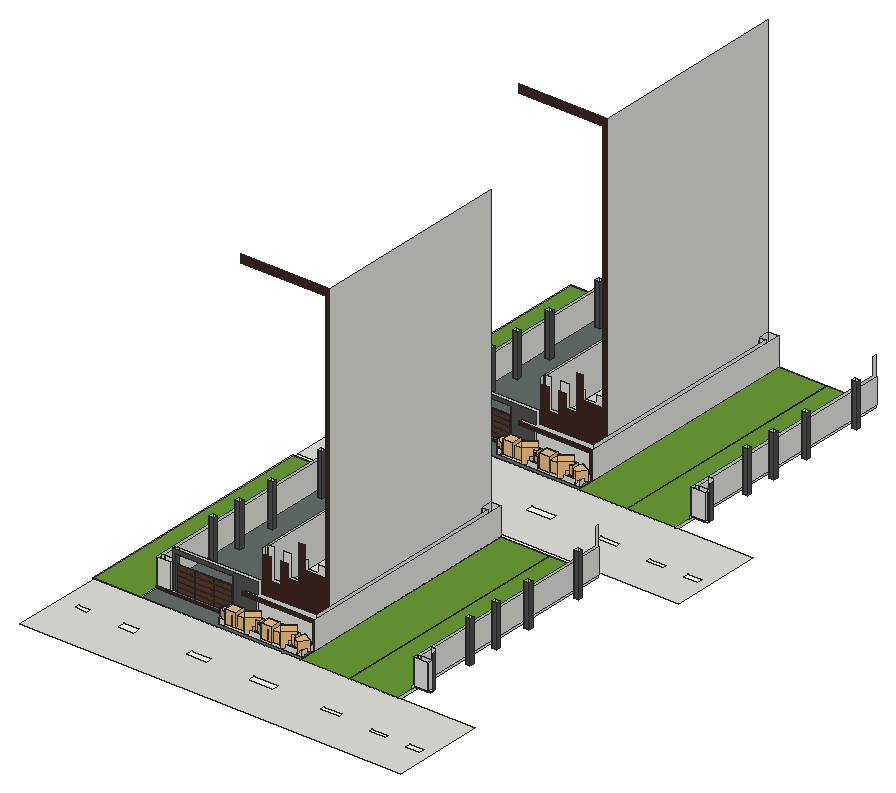
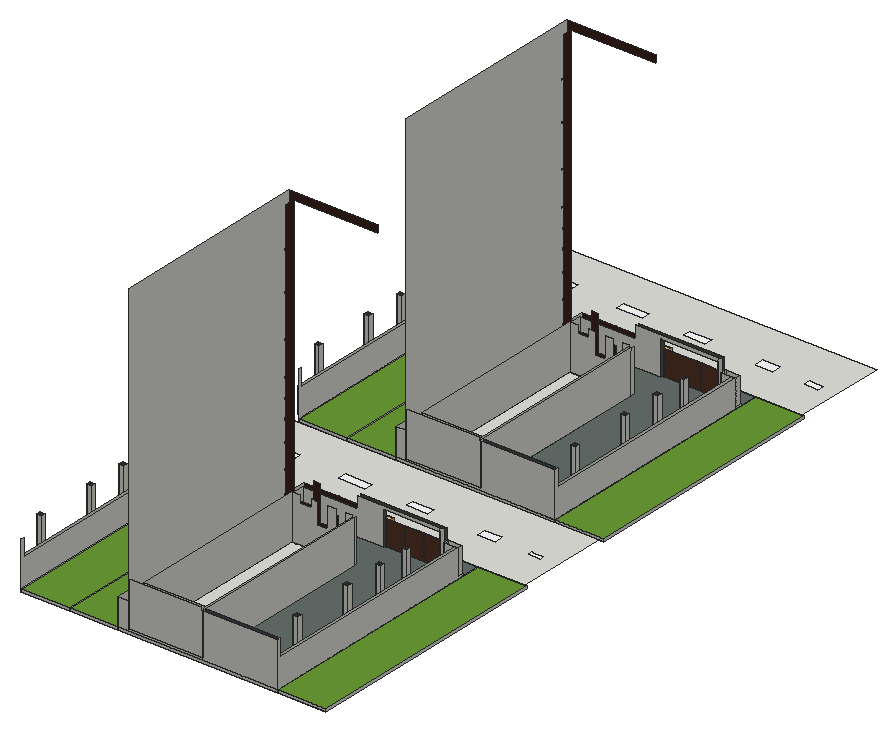
# SketchUp Ruby script. Lengths in inches.
U = 1.inch
M = Sketchup.active_model
def pt(a) = Geom::Point3d.new(a.map { |v| v * U })
def face(e, loops, mat)
  f = e.add_face(loops[0].map { |a| pt(a) })
  loops[1..].each { |l| e.add_face(l.map { |a| pt(a) }).erase! }
  f.material = f.back_material = mat if mat
  f
end
# faces: each face lists its corners as indices into pts; further lists are holes
def faces(e, pts, list, mat = nil) = list.each { |f| face(e, (f[0].is_a?(Array) ? f : [f]).map { |l| l.map { |i| pts[i] } }, mat) }
# xy, xz, yz: faces in a plane at the given z, y or x. An outline is a flat list of corners, or four numbers for a rectangle; further outlines are holes
def ring(l) = l.size == 4 ? [[l[0], l[1]], [l[2], l[1]], [l[2], l[3]], [l[0], l[3]]] : l.each_slice(2).to_a
def flat(e, list, mat, &to3) = list.each { |f| face(e, (f[0].is_a?(Array) ? f : [f]).map { |l| ring(l).map { |u, v| to3.(u, v) } }, mat) }
def xy(e, z, list, mat = nil) = flat(e, list, mat) { |x, y| [x, y, z] }
def xz(e, y, list, mat = nil) = flat(e, list, mat) { |x, z| [x, y, z] }
def yz(e, x, list, mat = nil) = flat(e, list, mat) { |y, z| [x, y, z] }
def lines(e, pts, list) = list.each { |a, b| e.add_line(pt(pts[a]), pt(pts[b])) }
# prism: a flat outline (further loops are holes) pulled along v
def prism(e, loops, v, mat = nil)
  f = face(e, loops, mat); d = Geom::Vector3d.new(v.map { |x| x * U })
  f.pushpull(f.normal.samedirection?(d) ? d.length : -d.length)
end
def box(e, o, s, mat = nil) = prism(e, [[o, [o[0] + s[0], o[1], o[2]], [o[0] + s[0], o[1] + s[1], o[2]], [o[0], o[1] + s[1], o[2]]]], [0, 0, s[2]], mat)
def at(x, y, z, deg = 0) = Geom::Transformation.translation(pt([x, y, z])) * Geom::Transformation.rotation(ORIGIN, Z_AXIS, deg.degrees)
def axes(o, x, y, z) = Geom::Transformation.new([*x, 0, *y, 0, *z, 0, *pt(o).to_a, 1])
def part(name) = M.definitions.add(name)
# library, detail: a bought-in or finely detailed component or shape, given as its bounding box
def library(name, o, s) = part(name).tap { |d| box(d.entities, o, s) }
def detail(e, o, s) = box(e.add_group.entities, o, s)
def put(e, d, t, mat = nil) = e.add_instance(d, t).tap { |i| i.material = mat if mat }
def group(e, t, mat = nil) = e.add_group.tap { |g| g.transformation = t; g.material = mat if mat }.entities
root = M.entities
M.materials.add("Color_").color = [255, 255, 255]
M.materials.add("Material__1").color = [95, 70, 46]
M.materials.add("[0043_SaddleBrown]").color = [63, 38, 31]
M.materials.add("[0135_DarkGray]").color = [81, 81, 81]
M.materials.add("[Color L16]").color = [51, 38, 20]
M.materials.add("[Formica Blue]").color = [73, 80, 86]
M.materials.add("[Grass Dark Green]").color = [105, 155, 54]
M.materials.add("[Slate]").color = [102, 110, 108]
M.materials.add("[Wood Veneer 01]").color = [89, 56, 41]
c1 = part("Grupo\#4")
xy(c1.entities,0,[[0,0,0,3.15,255.91,3.15,255.91,0,171.65,0,171.65,1.57,171.26,1.57,171.26,0,86.22,0,86.22,1.57,85.83,1.57,85.83,0]],"[Wood Veneer 01]")
xy(c1.entities,23.68,[[0,0,85.83,1.57],[86.22,0,171.26,1.57],[171.65,0,186.61,1.57],[186.61,0,255.91,1.57]],"[Color L16]")
xy(c1.entities,24.07,[[0,0,85.83,1.57],[86.22,0,168.11,1.57],[168.11,0,171.26,1.57],[171.65,0,255.91,1.57]],"[Color L16]")
xy(c1.entities,47.3,[[0,0,85.83,1.57],[86.22,0,89.76,1.57],[89.76,0,171.26,1.57],[171.65,0,255.91,1.57]],"[Color L16]")
xy(c1.entities,47.69,[[0,0,85.83,1.57],[86.22,0,171.26,1.57],[171.65,0,255.91,1.57]],"[Color L16]")
xy(c1.entities,70.92,[[0,0,85.83,1.57],[86.22,0,171.26,1.57],[171.65,0,255.91,1.57]],"[Color L16]")
xy(c1.entities,71.3125,[[0,0,85.83,1.57],[86.22,0,171.26,1.57],[171.65,0,255.91,1.57]],"[Color L16]")
xy(c1.entities,94.54,[[0,0,85.83,1.57],[86.22,0,171.26,1.57],[171.65,0,255.91,1.57]],"[Color L16]")
xy(c1.entities,94.9375,[[0,0,85.83,1.57],[86.22,0,171.26,1.57],[171.65,0,255.91,1.57]],"[Color L16]")
xy(c1.entities,118.16,[[0,0,85.83,0,85.83,1.57,86.22,1.57,86.22,0,171.26,0,171.26,1.57,171.65,1.57,171.65,0,255.91,0,255.91,3.15,0,3.15]],"[Wood Veneer 01]")
xz(c1.entities,0,[[0,0,85.83,23.68],[86.22,0,171.26,23.68],[171.65,0,255.91,23.68],[0,24.07,85.83,47.3],[86.22,24.07,171.26,47.3],
  [171.65,24.07,255.91,47.3],[0,47.69,85.83,70.92],[86.22,47.69,171.26,70.92],[171.65,47.69,255.91,70.92],[0,71.3125,85.83,94.54],
  [86.22,71.3125,171.26,94.54],[171.65,71.3125,255.91,94.54],[0,94.9375,85.83,118.16],[86.22,94.9375,171.26,118.16],[171.65,94.9375,255.91,118.16]],"[Wood Veneer 01]")
xz(c1.entities,1.57,[[[85.83,0,86.22,0,86.22,23.68,171.26,23.68,171.26,0,171.65,0,171.65,23.68,255.91,23.68,255.91,24.07,171.65,24.07,171.65,47.3,255.91,47.3,255.91,47.69,171.65,47.69,171.65,70.92,255.91,70.92,255.91,71.3125,171.65,71.3125,171.65,94.54,255.91,94.54,255.91,94.9375,171.65,94.9375,171.65,118.16,171.26,118.16,171.26,94.9375,86.22,94.9375,86.22,118.16,85.83,118.16,85.83,94.9375,0,94.9375,0,94.54,85.83,94.54,85.83,71.3125,0,71.3125,0,70.92,85.83,70.92,85.83,47.69,0,47.69,0,47.3,85.83,47.3,85.83,24.07,0,24.07,0,23.68,85.83,23.68],[86.22,71.3125,171.26,94.54],[86.22,24.07,171.26,47.3],[86.22,47.69,171.26,70.92]]],"[Color L16]")
xz(c1.entities,3.15,[[0,0,255.91,118.16]],"[Wood Veneer 01]")
yz(c1.entities,0,[[0,0,0,23.68,1.57,23.68,1.57,24.07,0,24.07,0,47.3,1.57,47.3,1.57,47.69,0,47.69,0,70.92,1.57,70.92,1.57,71.3125,0,71.3125,0,94.54,1.57,94.54,1.57,94.9375,0,94.9375,0,118.16,3.15,118.16,3.15,0]],"[Wood Veneer 01]")
yz(c1.entities,85.83,[[0,0,1.57,23.68],[0,24.07,1.57,47.3],[0,47.69,1.57,70.92],[0,71.3125,1.57,94.54],[0,94.9375,1.57,118.16]],"[Color L16]")
yz(c1.entities,86.22,[[0,0,1.57,23.68],[0,24.07,1.57,47.3],[0,47.69,1.57,70.92],[0,71.3125,1.57,94.54],[0,94.9375,1.57,118.16]],"[Color L16]")
yz(c1.entities,171.26,[[0,0,1.57,23.68],[0,24.07,1.57,47.3],[0,47.69,1.57,70.92],[0,71.3125,1.57,94.54],[0,94.9375,1.57,118.16]],"[Color L16]")
yz(c1.entities,171.65,[[0,0,1.57,23.68],[0,24.07,1.57,47.3],[0,47.69,1.57,70.92],[0,71.3125,1.57,94.54],[0,94.9375,1.57,118.16]],"[Color L16]")
yz(c1.entities,255.91,[[0,0,3.15,0,3.15,118.16,0,118.16,0,94.9375,1.57,94.9375,1.57,94.54,0,94.54,0,71.3125,1.57,71.3125,1.57,70.92,0,70.92,0,47.69,1.57,47.69,1.57,47.3,0,47.3,0,24.07,1.57,24.07,1.57,23.68,0,23.68]],"[Wood Veneer 01]")
c2 = library("Areca palm plant",[0,0,0],[49.1,36.6,54.46])
c3 = library("Group\#331",[-7.34,-1.2,0],[38.67,35.81,49.04])
c4 = library("Group38\#2",[14.01,28.44,-23.43],[18.58,18.32,38.89])
c5 = library("Group\#330",[-84.69,-90.07,-0.36],[176.51,175.13,171.4])
c6 = library("Group20\#1",[-20.81,-17.08,3.79],[39.86,39.43,37.51])
c7 = part("Group\#333")
put(c7.entities,c2,axes([-6.2,158.41,6.08],[0.45017,-0.56191,0],[0.66137,0.52986,0],[0,0,0.72]))
put(c7.entities,c2,axes([-6.2,56.6,6.08],[0.45017,-0.56191,0],[0.66137,0.52986,0],[0,0,0.72]))
put(c7.entities,c3,axes([24.9375,191.72,8],[0,0.79,0],[-0.79,0,0],[0,0,0.79]))
put(c7.entities,c4,axes([-4.1,100.66,28.17],[0.8848,0,0],[0,0.94674,0],[0,0,0.85826]))
g1 = group(c7.entities,at(0,0,0))
xy(g1,0,[[0,0,6,234.8],[30,0,36,234.8]])
xy(g1,3,[[6,0,30,234.8]])
xy(g1,7,[[6,5,30,229.8]],"Material__1")
xy(g1,15,[[[0,0,36,234.8],[6,5,30,229.8]]])
xz(g1,0,[[0,0,6,0,6,3,30,3,30,0,36,0,36,15,0,15]])
xz(g1,5,[[6,7,30,15]])
xz(g1,229.8,[[6,7,30,15]])
xz(g1,234.8,[[0,0,0,15,36,15,36,0,30,0,30,3,6,3,6,0]])
yz(g1,0,[[0,0,234.8,15]])
yz(g1,6,[[0,0,234.8,3],[5,7,229.8,15]])
yz(g1,30,[[0,0,234.8,3],[5,7,229.8,15]])
yz(g1,36,[[0,0,234.8,15]])
put(c7.entities,c5,axes([17.19,223.04,6.07],[-0.08133,-0.14087,0],[0.14087,-0.08133,0],[0,0,0.1725]))
put(c7.entities,c6,axes([18.97,181.79,4.77],[0,0.85,0],[-0.85,0,0],[0,0,0.85]))
put(c7.entities,c3,axes([24.9375,89.91,8],[0,0.79,0],[-0.79,0,0],[0,0,0.79]))
put(c7.entities,c4,axes([-4.1,-1.15,28.17],[0.8848,0,0],[0,0.94674,0],[0,0,0.85826]))
put(c7.entities,c5,axes([17.19,121.23,6.07],[-0.08133,-0.14087,0],[0.14087,-0.08133,0],[0,0,0.1725]))
put(c7.entities,c5,axes([14.93,91.37,6.05],[-0.04961,-0.08593,0],[0.08593,-0.04961,0],[0,0,0.10522]))
put(c7.entities,c5,axes([17.19,15.79,6.07],[-0.08133,-0.14087,0],[0.14087,-0.08133,0],[0,0,0.1725]))
put(c7.entities,c6,axes([18.97,79.98,4.77],[0,0.85,0],[-0.85,0,0],[0,0,0.85]))
put(c7.entities,c5,axes([14.93,44.05,6.05],[-0.04961,-0.08593,0],[0.08593,-0.04961,0],[0,0,0.10522]))
put(c7.entities,c5,axes([14.93,71.3,6.05],[-0.04961,-0.08593,0],[0.08593,-0.04961,0],[0,0,0.10522]))
put(c7.entities,c5,axes([14.93,173.12,6.05],[-0.04961,-0.08593,0],[0.08593,-0.04961,0],[0,0,0.10522]))
put(c7.entities,c5,axes([14.93,193.18,6.05],[-0.04961,-0.08593,0],[0.08593,-0.04961,0],[0,0,0.10522]))
put(c7.entities,c5,axes([14.93,145.87,6.05],[-0.04961,-0.08593,0],[0.08593,-0.04961,0],[0,0,0.10522]))
c8 = part("Untitled (5)")
xy(c8.entities,0,[[[158.81,26.5625,306.06,993.3125],[226.57,518.17,239.57,583.92],[225.28,357.51,237.28,411.51],[222.61,182.28,236.36,226.53],[239.71,931.55,251.46,972.3],[233.64,703.93,242.14,755.18],[240.05,835.03,248.8,880.53],[222.04,66.5,231.29,100.5]]])
xy(c8.entities,0,[[222.04,66.5,231.29,100.5],[222.61,182.28,236.36,226.53],[225.28,357.51,237.28,411.51],[226.57,518.17,239.57,583.92],[233.64,703.93,242.14,755.18],
  [240.05,835.03,248.8,880.53],[239.71,931.55,251.46,972.3]],"Color_")
xy(root,-7.1875,[[0,272.41,137.5,980.35],[137.5,272.41,586.9375,980.35],[586.9375,272.41,724.4375,980.35],[724.4375,272.41,861.9375,980.35],[0,1252.76,137.5,1960.7],
  [137.5,1252.76,586.9375,1960.7],[586.9375,1252.76,724.4375,1960.7],[724.4375,1252.76,861.9375,1960.7]])
xy(root,0,[[137.5,324.35,586.9375,980.35],[137.5,1304.7,586.9375,1960.7]])
xy(root,0,[[0,272.41,137.5,980.35],[586.9375,272.41,724.4375,980.35],[724.4375,272.41,861.9375,980.35],[0,1252.76,137.5,1960.7],[586.9375,1252.76,724.4375,1960.7],
  [724.4375,1252.76,861.9375,1960.7]],"[Grass Dark Green]")
xy(root,0,[[137.5,272.41,586.9375,324.35],[137.5,1252.76,586.9375,1304.7]],"[Slate]")
xy(root,6.125,[[137.5,324.35,177.74,328.54],[177.74,324.35,188.43,332.35],[861.9375,324.35,902.18,328.54],[902.18,324.35,912.87,332.35],[137.5,328.54,177.74,343.16],
  [861.9375,328.54,902.18,343.16],[[547.05,412.04,547.05,438.72,348.1875,438.72,348.1875,980.35,558.625,980.35,558.625,412.04],[353.97,447.84,521.63,971.23]],[353.97,447.84,521.63,971.23],[166.95,475.13,180.58,487.19],[891.39,475.13,905.02,487.19],
  [166.95,567.38,180.58,579.44],[891.39,567.38,905.02,579.44],[166.95,682.44,180.58,694.5],[891.39,682.44,905.02,694.5],[166.95,858.25,180.58,870.31],
  [891.39,858.25,905.02,870.31],[137.5,1304.7,177.74,1308.89],[177.74,1304.7,188.43,1312.7],[861.9375,1304.7,902.18,1308.89],[902.18,1304.7,912.87,1312.7],
  [137.5,1308.89,177.74,1323.51],[861.9375,1308.89,902.18,1323.51],[[547.05,1392.39,547.05,1419.07,348.1875,1419.07,348.1875,1960.7,558.625,1960.7,558.625,1392.39],[353.97,1428.19,521.63,1951.58]],[353.97,1428.19,521.63,1951.58],[166.95,1455.48,180.58,1467.54],
  [891.39,1455.48,905.02,1467.54],[166.95,1547.73,180.58,1559.79],[891.39,1547.73,905.02,1559.79],[166.95,1662.79,180.58,1674.85],[891.39,1662.79,905.02,1674.85],
  [166.95,1838.6,180.58,1850.66],[891.39,1838.6,905.02,1850.66]])
xy(root,6.125,[[[188.43,324.35,348.44,324.35,348.44,341.79,577.26,341.79,577.26,948.22,558.625,948.22,558.625,412.04,547.05,412.04,547.05,438.72,348.1875,438.72,348.1875,971.23,146.62,971.23,146.62,343.16,177.74,343.16,177.74,341.79,188.43,341.79],[166.95,858.25,180.58,870.31],[166.95,682.44,180.58,694.5],[166.95,567.38,180.58,579.44],[166.95,475.13,180.58,487.19]],[[188.43,1304.7,348.44,1304.7,348.44,1322.14,577.26,1322.14,577.26,1928.57,558.625,1928.57,558.625,1392.39,547.05,1392.39,547.05,1419.07,348.1875,1419.07,348.1875,1951.58,146.62,1951.58,146.62,1323.51,177.74,1323.51,177.74,1322.14,188.43,1322.14],[166.95,1838.6,180.58,1850.66],[166.95,1662.79,180.58,1674.85],[166.95,1547.73,180.58,1559.79],[166.95,1455.48,180.58,1467.54]]],"[Slate]")
xy(root,6.16,[[348.44,324.35,420.26,332.35],[348.44,1304.7,420.26,1312.7]])
xz(root,272.41,[[0,-7.1875,137.5,0],[137.5,-7.1875,586.9375,0],[586.9375,-7.1875,724.4375,0],[724.4375,-7.1875,861.9375,0]])
xz(root,324.35,[[137.5,0,586.9375,0,586.9375,77.97,379.07,77.97,379.07,67.07,580.26,67.07,580.26,14.13,420.26,14.13,420.26,6.16,348.44,6.16,348.44,6.125,137.5,6.125]],"[0043_SaddleBrown]")
xz(root,328.54,[[137.5,6.125,177.74,77.97],[861.9375,6.125,902.18,77.97]])
xz(root,332.35,[[177.74,6.125,188.43,6.125,188.43,102.02,348.44,102.02,348.44,6.16,420.26,6.16,420.26,67.07,379.07,67.07,379.07,77.97,420.26,77.97,420.26,111.97,177.74,111.97]],"[0135_DarkGray]")
xz(root,341.79,[[177.74,6.125,188.43,111.97],[348.44,6.125,348.44,102.02,188.43,102.02,188.43,111.97,420.26,111.97,420.26,77.97,577.26,77.97,577.26,6.125],[902.18,6.125,912.87,111.97]])
xz(root,343.16,[[137.5,6.125,146.62,77.97],[146.62,6.125,177.74,77.97],[861.9375,6.125,871.06,77.97],[871.06,6.125,902.18,77.97]])
xz(root,412.04,[[547.05,6.125,558.625,6.125,558.625,866.5625,308.59,866.5625,308.59,845.41,547.05,845.41]],"[0043_SaddleBrown]")
xz(root,447.84,[[353.97,6.125,353.97,132.25,370.54,132.25,370.54,50.14,399.16,50.14,399.16,132.25,419.76,132.25,419.76,73.83,451.01,73.83,451.01,132.25,467.3,132.25,467.3,110.73,500.42,110.73,500.42,132.25,521.63,132.25,521.63,6.125]])
xz(root,475.13,[[166.95,6.125,180.58,126.125],[891.39,6.125,905.02,126.125]],"[0135_DarkGray]")
xz(root,487.19,[[166.95,6.125,180.58,126.125],[891.39,6.125,905.02,126.125]])
xz(root,567.38,[[166.95,6.125,180.58,126.125],[891.39,6.125,905.02,126.125]],"[0135_DarkGray]")
xz(root,579.44,[[166.95,6.125,180.58,126.125],[891.39,6.125,905.02,126.125]])
xz(root,682.44,[[166.95,6.125,180.58,126.125],[891.39,6.125,905.02,126.125]],"[0135_DarkGray]")
xz(root,694.5,[[166.95,6.125,180.58,126.125],[891.39,6.125,905.02,126.125]])
xz(root,858.25,[[166.95,6.125,180.58,126.125],[891.39,6.125,905.02,126.125]],"[0135_DarkGray]")
xz(root,870.31,[[166.95,6.125,180.58,126.125],[891.39,6.125,905.02,126.125]])
xz(root,948.22,[[558.625,6.125,577.26,77.97]])
xz(root,971.23,[[353.97,6.125,521.63,132.25]])
xz(root,971.23,[[146.62,6.125,348.1875,126.125]],"[Formica Blue]")
xz(root,980.35,[[0,-7.1875,137.5,0],[137.5,-7.1875,586.9375,0],[586.9375,-7.1875,724.4375,0],[724.4375,-7.1875,861.9375,0],[137.5,0,137.5,126.125,348.1875,126.125,348.1875,6.125,558.625,6.125,558.625,77.97,586.9375,77.97,586.9375,0],
  [348.1875,6.125,348.1875,126.125,353.97,126.125,353.97,132.25,558.625,132.25,558.625,6.125]])
xz(root,1252.76,[[0,-7.1875,137.5,0],[137.5,-7.1875,586.9375,0],[586.9375,-7.1875,724.4375,0],[724.4375,-7.1875,861.9375,0]])
xz(root,1304.7,[[137.5,0,586.9375,0,586.9375,77.97,379.07,77.97,379.07,67.07,580.26,67.07,580.26,14.13,420.26,14.13,420.26,6.16,348.44,6.16,348.44,6.125,137.5,6.125]],"[0043_SaddleBrown]")
xz(root,1308.89,[[137.5,6.125,177.74,77.97],[861.9375,6.125,902.18,77.97]])
xz(root,1312.7,[[177.74,6.125,188.43,6.125,188.43,102.02,348.44,102.02,348.44,6.16,420.26,6.16,420.26,67.07,379.07,67.07,379.07,77.97,420.26,77.97,420.26,111.97,177.74,111.97]],"[0135_DarkGray]")
xz(root,1322.14,[[177.74,6.125,188.43,111.97],[348.44,6.125,348.44,102.02,188.43,102.02,188.43,111.97,420.26,111.97,420.26,77.97,577.26,77.97,577.26,6.125],[902.18,6.125,912.87,111.97]])
xz(root,1323.51,[[137.5,6.125,146.62,77.97],[146.62,6.125,177.74,77.97],[861.9375,6.125,871.06,77.97],[871.06,6.125,902.18,77.97]])
xz(root,1392.39,[[547.05,6.125,558.625,6.125,558.625,866.5625,308.59,866.5625,308.59,845.41,547.05,845.41]],"[0043_SaddleBrown]")
xz(root,1428.19,[[353.97,6.125,353.97,132.25,370.54,132.25,370.54,50.14,399.16,50.14,399.16,132.25,419.76,132.25,419.76,73.83,451.01,73.83,451.01,132.25,467.3,132.25,467.3,110.73,500.42,110.73,500.42,132.25,521.63,132.25,521.63,6.125]])
xz(root,1455.48,[[166.95,6.125,180.58,126.125],[891.39,6.125,905.02,126.125]],"[0135_DarkGray]")
xz(root,1467.54,[[166.95,6.125,180.58,126.125],[891.39,6.125,905.02,126.125]])
xz(root,1547.73,[[166.95,6.125,180.58,126.125],[891.39,6.125,905.02,126.125]],"[0135_DarkGray]")
xz(root,1559.79,[[166.95,6.125,180.58,126.125],[891.39,6.125,905.02,126.125]])
xz(root,1662.79,[[166.95,6.125,180.58,126.125],[891.39,6.125,905.02,126.125]],"[0135_DarkGray]")
xz(root,1674.85,[[166.95,6.125,180.58,126.125],[891.39,6.125,905.02,126.125]])
xz(root,1838.6,[[166.95,6.125,180.58,126.125],[891.39,6.125,905.02,126.125]],"[0135_DarkGray]")
xz(root,1850.66,[[166.95,6.125,180.58,126.125],[891.39,6.125,905.02,126.125]])
xz(root,1928.57,[[558.625,6.125,577.26,77.97]])
xz(root,1951.58,[[353.97,6.125,521.63,132.25]])
xz(root,1951.58,[[146.62,6.125,348.1875,126.125]],"[Formica Blue]")
xz(root,1960.7,[[0,-7.1875,137.5,0],[137.5,-7.1875,586.9375,0],[586.9375,-7.1875,724.4375,0],[724.4375,-7.1875,861.9375,0],[137.5,0,137.5,126.125,348.1875,126.125,348.1875,6.125,558.625,6.125,558.625,77.97,586.9375,77.97,586.9375,0],
  [348.1875,6.125,348.1875,126.125,353.97,126.125,353.97,132.25,558.625,132.25,558.625,6.125]])
yz(root,0,[[272.41,-7.1875,980.35,0],[1252.76,-7.1875,1960.7,0]])
yz(root,137.5,[[272.41,-7.1875,980.35,0],[1252.76,-7.1875,1960.7,0],[324.35,0,324.35,6.125,343.16,6.125,343.16,77.97,971.23,77.97,971.23,126.125,980.35,126.125,980.35,0],[1304.7,0,1304.7,6.125,1323.51,6.125,1323.51,77.97,1951.58,77.97,1951.58,126.125,1960.7,126.125,1960.7,0],[328.54,6.125,343.16,77.97],
  [1308.89,6.125,1323.51,77.97]])
yz(root,146.62,[[343.16,6.125,971.23,77.97],[1323.51,6.125,1951.58,77.97]])
yz(root,166.95,[[475.13,6.125,487.19,126.125],[567.38,6.125,579.44,126.125],[682.44,6.125,694.5,126.125],[858.25,6.125,870.31,126.125],[1455.48,6.125,1467.54,126.125],
  [1547.73,6.125,1559.79,126.125],[1662.79,6.125,1674.85,126.125],[1838.6,6.125,1850.66,126.125]])
yz(root,177.74,[[328.54,6.125,332.35,77.97],[332.35,6.125,341.79,77.97],[341.79,6.125,343.16,77.97],[1308.89,6.125,1312.7,77.97],[1312.7,6.125,1322.14,77.97],
  [1322.14,6.125,1323.51,77.97]])
yz(root,180.58,[[475.13,6.125,487.19,126.125],[567.38,6.125,579.44,126.125],[682.44,6.125,694.5,126.125],[858.25,6.125,870.31,126.125],[1455.48,6.125,1467.54,126.125],
  [1547.73,6.125,1559.79,126.125],[1662.79,6.125,1674.85,126.125],[1838.6,6.125,1850.66,126.125]],"[0135_DarkGray]")
yz(root,188.43,[[332.35,6.125,341.79,102.02],[1312.7,6.125,1322.14,102.02]],"[0135_DarkGray]")
yz(root,348.1875,[[438.72,6.125,438.72,109.76,441.04,109.76,441.04,112.41,438.72,112.41,438.72,126.125,447.84,126.125,447.84,6.125],[447.84,6.125,971.23,126.125],[971.23,6.125,980.35,126.125],[1419.07,6.125,1419.07,109.76,1421.39,109.76,1421.39,112.41,1419.07,112.41,1419.07,126.125,1428.19,126.125,1428.19,6.125],[1428.19,6.125,1951.58,126.125],
  [1951.58,6.125,1960.7,126.125]])
yz(root,348.44,[[324.35,6.125,324.35,6.16,332.35,6.16,332.35,102.02,341.79,102.02,341.79,6.125],[1304.7,6.125,1304.7,6.16,1312.7,6.16,1312.7,102.02,1322.14,102.02,1322.14,6.125]],"[0135_DarkGray]")
yz(root,353.97,[[447.84,6.125,971.23,126.125],[1428.19,6.125,1951.58,126.125]])
yz(root,420.26,[[324.35,6.16,324.35,14.13,328.54,14.13,328.54,67.07,332.35,67.07,332.35,6.16],[1304.7,6.16,1304.7,14.13,1308.89,14.13,1308.89,67.07,1312.7,67.07,1312.7,6.16]])
yz(root,521.63,[[447.84,6.125,971.23,132.25],[1428.19,6.125,1951.58,132.25]])
yz(root,547.05,[[412.04,6.125,412.04,845.41,438.72,845.41,438.73,736,442.66,736,442.66,733.125,438.72,733.125,438.73,626.6,442.66,626.6,442.66,623.5625,438.73,623.5625,438.73,508.42,442.66,508.42,442.66,505.6875,438.73,505.6875,438.73,412.48,442.66,412.48,442.66,409.48,438.73,409.48,438.73,357.3,441.04,357.3,441.04,354.27,438.72,354.27,438.72,306.7,441.04,306.7,441.04,303,438.73,303,438.73,246.28,441.04,246.28,441.04,243.96,438.73,243.96,438.73,177.22,441.04,177.22,441.04,174.81,438.73,174.81,438.73,114.29,441.04,114.29,441.04,110.73,438.72,110.73,438.72,6.125],[1392.39,6.125,1392.39,845.41,1419.07,845.41,1419.08,736,1423.01,736,1423.01,733.125,1419.07,733.125,1419.08,626.6,1423.01,626.6,1423.01,623.5625,1419.08,623.5625,1419.08,508.42,1423.01,508.42,1423.01,505.6875,1419.08,505.6875,1419.08,412.48,1423.01,412.48,1423.01,409.48,1419.08,409.48,1419.08,357.3,1421.39,357.3,1421.39,354.27,1419.07,354.27,1419.07,306.7,1421.39,306.7,1421.39,303,1419.08,303,1419.08,246.28,1421.39,246.28,1421.39,243.96,1419.08,243.96,1419.08,177.22,1421.39,177.22,1421.39,174.81,1419.08,174.81,1419.08,114.29,1421.39,114.29,1421.39,110.73,1419.07,110.73,1419.07,6.125]],"[0043_SaddleBrown]")
yz(root,558.625,[[412.04,6.125,948.22,6.125,948.22,77.97,980.35,77.97,980.35,866.5625,412.04,866.5625],[948.22,6.125,980.35,77.97],[1392.39,6.125,1928.57,6.125,1928.57,77.97,1960.7,77.97,1960.7,866.5625,1392.39,866.5625],[1928.57,6.125,1960.7,77.97]])
yz(root,577.26,[[341.79,6.125,948.22,77.97],[1322.14,6.125,1928.57,77.97]])
yz(root,586.9375,[[272.41,-7.1875,980.35,0],[1252.76,-7.1875,1960.7,0],[324.35,0,980.35,77.97],[1304.7,0,1960.7,77.97]])
yz(root,724.4375,[[272.41,-7.1875,980.35,0],[1252.76,-7.1875,1960.7,0]])
yz(root,861.9375,[[272.41,-7.1875,980.35,0],[1252.76,-7.1875,1960.7,0],[324.35,0,324.35,6.125,343.16,6.125,343.16,77.97,971.23,77.97,971.23,126.125,980.35,126.125,980.35,0],[1304.7,0,1304.7,6.125,1323.51,6.125,1323.51,77.97,1951.58,77.97,1951.58,126.125,1960.7,126.125,1960.7,0],[328.54,6.125,343.16,77.97],
  [1308.89,6.125,1323.51,77.97]])
yz(root,871.06,[[343.16,6.125,971.23,77.97],[1323.51,6.125,1951.58,77.97]])
yz(root,891.39,[[475.13,6.125,487.19,126.125],[567.38,6.125,579.44,126.125],[682.44,6.125,694.5,126.125],[858.25,6.125,870.31,126.125],[1455.48,6.125,1467.54,126.125],
  [1547.73,6.125,1559.79,126.125],[1662.79,6.125,1674.85,126.125],[1838.6,6.125,1850.66,126.125]])
yz(root,902.18,[[328.54,6.125,332.35,77.97],[332.35,6.125,341.79,77.97],[341.79,6.125,343.16,77.97],[1308.89,6.125,1312.7,77.97],[1312.7,6.125,1322.14,77.97],
  [1322.14,6.125,1323.51,77.97]])
yz(root,905.02,[[475.13,6.125,487.19,126.125],[567.38,6.125,579.44,126.125],[682.44,6.125,694.5,126.125],[858.25,6.125,870.31,126.125],[1455.48,6.125,1467.54,126.125],
  [1547.73,6.125,1559.79,126.125],[1662.79,6.125,1674.85,126.125],[1838.6,6.125,1850.66,126.125]],"[0135_DarkGray]")
yz(root,912.87,[[332.35,6.125,341.79,102.02],[1312.7,6.125,1322.14,102.02]],"[0135_DarkGray]")
p = [[547.05,438.72,6.125],[547.05,438.72,110.73],[500.42,438.72,110.73],[467.3,438.72,110.73],[467.3,438.72,173.82],[451.01,438.72,173.82],
  [451.01,438.72,73.83],[419.76,438.72,73.83],[419.76,438.72,109.99],[399.16,438.73,109.99],[399.16,438.72,50.14],[370.54,438.72,50.14],
  [370.54,438.72,109.76],[348.1875,438.72,109.76],[348.1875,438.72,6.125],[547.05,1419.07,6.125],[547.05,1419.07,110.73],[500.42,1419.07,110.73],
  [467.3,1419.07,110.73],[467.3,1419.07,173.82],[451.01,1419.07,173.82],[451.01,1419.07,73.83],[419.76,1419.07,73.83],[419.76,1419.07,109.99],
  [399.16,1419.08,109.99],[399.16,1419.07,50.14],[370.54,1419.07,50.14],[370.54,1419.08,109.76],[348.1875,1419.07,109.76],[348.1875,1419.07,6.125]]
faces(root,p,[[0,1,2,3,4,5,6,7,8,9,10,11,12,13,14],[15,16,17,18,19,20,21,22,23,24,25,26,27,28,29]],"[0043_SaddleBrown]")
put(root,c1,axes([187.97,333.55,2.37],[0.6177,0,0],[0,0.6177,0],[0,0,0.6177]))
put(root,c1,axes([187.97,1313.9,2.37],[0.6177,0,0],[0,0.6177,0],[0,0,0.6177]))
put(root,c7,at(582.88,284.24,0,90))
put(root,c7,at(582.88,1264.59,0,90))
put(root,c8,axes([-23.97,555.32,0],[0,-1.78,0],[1.11229,0,0],[0,0,1]))
put(root,c8,axes([-23.97,1535.67,0],[0,-1.78,0],[1.11229,0,0],[0,0,1]))
